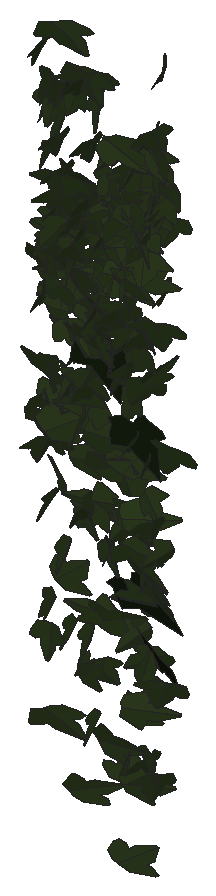
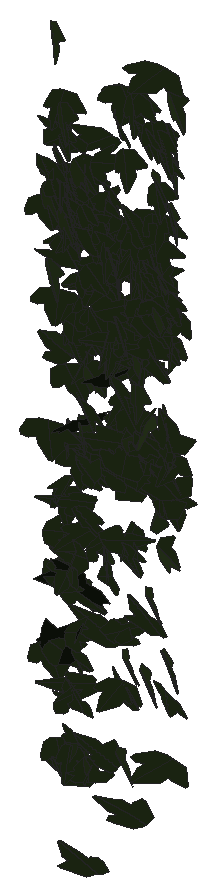
# SketchUp Ruby script. Lengths in millimetres.
U = 1.mm
M = Sketchup.active_model
def pt(a) = Geom::Point3d.new(a.map { |v| v * U })
def face(e, loops, mat)
  f = e.add_face(loops[0].map { |a| pt(a) })
  loops[1..].each { |l| e.add_face(l.map { |a| pt(a) }).erase! }
  f.material = f.back_material = mat if mat
  f
end
# faces: each face lists its corners as indices into pts; further lists are holes
def faces(e, pts, list, mat = nil) = list.each { |f| face(e, (f[0].is_a?(Array) ? f : [f]).map { |l| l.map { |i| pts[i] } }, mat) }
# xy, xz, yz: faces in a plane at the given z, y or x. An outline is a flat list of corners, or four numbers for a rectangle; further outlines are holes
def ring(l) = l.size == 4 ? [[l[0], l[1]], [l[2], l[1]], [l[2], l[3]], [l[0], l[3]]] : l.each_slice(2).to_a
def flat(e, list, mat, &to3) = list.each { |f| face(e, (f[0].is_a?(Array) ? f : [f]).map { |l| ring(l).map { |u, v| to3.(u, v) } }, mat) }
def xy(e, z, list, mat = nil) = flat(e, list, mat) { |x, y| [x, y, z] }
def xz(e, y, list, mat = nil) = flat(e, list, mat) { |x, z| [x, y, z] }
def yz(e, x, list, mat = nil) = flat(e, list, mat) { |y, z| [x, y, z] }
def lines(e, pts, list) = list.each { |a, b| e.add_line(pt(pts[a]), pt(pts[b])) }
# prism: a flat outline (further loops are holes) pulled along v
def prism(e, loops, v, mat = nil)
  f = face(e, loops, mat); d = Geom::Vector3d.new(v.map { |x| x * U })
  f.pushpull(f.normal.samedirection?(d) ? d.length : -d.length)
end
def box(e, o, s, mat = nil) = prism(e, [[o, [o[0] + s[0], o[1], o[2]], [o[0] + s[0], o[1] + s[1], o[2]], [o[0], o[1] + s[1], o[2]]]], [0, 0, s[2]], mat)
def at(x, y, z, deg = 0) = Geom::Transformation.translation(pt([x, y, z])) * Geom::Transformation.rotation(ORIGIN, Z_AXIS, deg.degrees)
def axes(o, x, y, z) = Geom::Transformation.new([*x, 0, *y, 0, *z, 0, *pt(o).to_a, 1])
def part(name) = M.definitions.add(name)
# library, detail: a bought-in or finely detailed component or shape, given as its bounding box
def library(name, o, s) = part(name).tap { |d| box(d.entities, o, s) }
def detail(e, o, s) = box(e.add_group.entities, o, s)
def put(e, d, t, mat = nil) = e.add_instance(d, t).tap { |i| i.material = mat if mat }
def group(e, t, mat = nil) = e.add_group.tap { |g| g.transformation = t; g.material = mat if mat }.entities
root = M.entities
M.materials.add("efeu1").color = [18, 25, 13]
M.materials.add("efeu2").color = [43, 57, 29]
c1 = part("ivyleaf_10")
p = [[0,12.8,-0.8],[-1.5,51.3,-10.9],[-4.9,51,-11.6],[-13.6,26.5,-7.3],[-13.2,15.9,-4.6],[-21.1,19.3,-7.2],
  [-29.5,16.3,-8.3],[-29.2,8.3,-6.2],[-19.7,-9.8,0.5],[-7.6,-13,4],[1,-12.2,5.8],[-0.4,51.1,-11.1],
  [-1.5,51.1,-10.9],[1,-12.4,5.9],[16.9,-12.4,3.5],[35.1,9.1,-5.1],[35,12.9,-6.1],[20.5,16.4,-4.9],
  [15.8,15,-3.8],[15.3,27.6,-7.1],[12.8,31.3,-7.8]]
faces(c1.entities,p,[[0,1,2,3,4,5,6,7,8,9,10],[11,12,0,13,14,15,16,17,18,19,20]],"efeu2")
c2 = part("ivyleaf_9")
p = [[39.1,54.8,31.7],[34.5,51.8,30.2],[-5.3,25.2,17.3],[-17.9,28.3,20.9],[-21.6,21.7,17],[-20.2,4.3,5.3],
  [-22.9,-0.3,2.5],[-17.1,-4,-0.6],[-2,-2.1,-1.2],[-0.7,-15.4,-10.1],[16.6,-22.3,-16.7],[21.1,-15.1,-12.5],
  [32.7,-10.7,-11],[46.1,-1.8,-6.6],[30.8,11.2,3.8]]
faces(c2.entities,p,[[0,1,2,3,4,5,6,7,8,9,10,11,12,13,14]],"efeu1")
put(root,c1,axes([1499.8,1027.3,1054.7],[0.18539,-0.72191,-0.0235],[-0.01929,0.02234,-0.72842],[1.37454,0.09768,-0.00705]))
put(root,c1,axes([1500.7,1029.5,518.1],[-0.35286,-0.6431,0.00823],[-0.00439,-0.0079,-0.66929],[1.22403,-0.18542,-0.00003]))
put(root,c1,axes([1490.9,1042.9,604],[-1.17234,0.16189,0.30669],[0.55873,-0.08938,0.63681],[0.35137,0.68228,0.01065]))
put(root,c1,axes([1501.9,1031.3,972.9],[0.35833,-0.62964,-0.25162],[-0.09136,0.24811,-0.65677],[1.28725,0.19288,0.02343]))
put(root,c1,axes([1493.9,1029.2,766.2],[-1.04653,0.28475,-0.17468],[0.27916,-0.09646,-0.61899],[-0.57121,-0.56884,0.01753]))
put(root,c1,axes([1502.7,1028.3,904.4],[0.33136,-0.59957,-0.27894],[-0.09067,0.27633,-0.62369],[1.25529,0.17823,0.02858]))
put(root,c1,axes([1496.4,1032.2,574.7],[-0.41017,-0.48565,-0.40585],[0.34836,0.36258,-0.53108],[1.15307,-0.2823,0.01608]))
put(root,c1,axes([1505.6,1032.9,304.2],[0.46916,-0.61543,-0.20288],[-0.14756,0.18749,-0.66296],[1.22442,0.25841,-0.00216]))
put(root,c1,axes([1504.6,1018,722.1],[-0.01377,-0.47935,-0.49437],[0.07307,0.49334,-0.47892],[1.30851,-0.03259,0.02154]))
put(root,c1,axes([1509.2,1046.3,787.9],[0.66422,0.37677,-0.38742],[-0.57736,-0.24507,-0.51163],[-0.85118,0.46025,0.04472]))
put(root,c1,axes([1507.2,1040.8,797.6],[1.1056,-0.27653,-0.19393],[-0.31433,0.10397,-0.643],[0.56071,0.60354,0.02192]))
put(root,c1,axes([1493.6,1040.6,538.2],[-0.81421,-0.42933,0.34425],[0.49786,0.22496,0.60565],[-0.92143,0.50092,0.02305]))
put(root,c1,axes([1509.2,1021,1005.8],[0.42926,-0.59634,-0.35365],[-0.15389,0.34673,-0.63624],[1.31052,0.23604,0.04113]))
put(root,c1,axes([1506.3,1041,826],[0.25976,-0.64431,0.12548],[0.02698,-0.12524,-0.6585],[1.24899,0.13671,-0.01187]))
put(root,c1,axes([1495.7,1044.8,513.9],[-0.98982,0.25845,0.41449],[0.69298,-0.19845,0.58062],[0.61968,0.63475,0.01276]))
put(root,c1,axes([1511.6,1032.1,1000.4],[0.67253,-0.44125,-0.43697],[-0.2608,0.43497,-0.55004],[1.15276,0.35584,0.13049]))
put(root,c1,axes([1523.8,1027.1,733.8],[-0.90524,0.162,0.39647],[-0.78739,-0.02057,-0.48794],[-0.2108,-0.61887,0.12]))
put(root,c1,axes([1500,1033.3,573.8],[-0.29107,0.53976,-0.39567],[0.21426,-0.37934,-0.56099],[-1.25557,-0.18986,-0.00401]))
put(root,c1,axes([1499.8,1037.6,258.7],[1.01907,-0.34827,0.22096],[0.35185,-0.12102,-0.63875],[0.7017,0.56647,-0.00062]))
put(root,c1,axes([1508.7,1044.1,775.6],[0.15782,-0.59778,0.32093],[0.14329,-0.31322,-0.60286],[1.28332,0.10849,0.02785]))
put(root,c1,axes([1530.7,1028.5,533.9],[-0.26969,0.05142,0.62374],[-1.13648,0.18037,-0.15053],[-0.35662,-0.61367,0.00802]))
put(root,c1,axes([1522,1016.5,613],[-0.01044,-0.01778,0.68873],[-0.81153,0.54108,0.01057],[-1.02993,-0.42616,-0.01531]))
put(root,c1,axes([1511,1032,448.2],[0.28195,-0.54853,0.36991],[0.13113,-0.36422,-0.56768],[1.25231,0.16164,-0.02384]))
put(root,c1,axes([1511.8,1043.3,947.8],[0.61311,-0.60836,0.03694],[0.05906,-0.02536,-0.68821],[1.15845,0.32327,0.01554]))
put(root,c1,axes([1534,1037.7,559.6],[-0.87151,-0.06403,0.53508],[-0.98256,-0.14922,-0.45968],[0.29409,-0.68828,0.04988]))
put(root,c1,axes([1508,1034.8,980.9],[1.05257,-0.41382,0.16129],[0.23218,-0.10614,-0.69064],[0.81279,0.56623,-0.01158]))
put(root,c1,axes([1517.6,1034.9,930.2],[-0.17866,-0.66963,-0.14527],[0.04485,0.14338,-0.67617],[1.30332,-0.09673,0.00336]))
put(root,c1,axes([1498.7,1045.9,584.6],[0.08546,-0.11336,0.64522],[0.93209,-0.42372,-0.10853],[0.82806,0.48865,0.05557]))
put(root,c1,axes([1520.2,1046.3,816],[1.13958,-0.12566,-0.22355],[-0.4224,0.03057,-0.61164],[0.24454,0.63841,-0.01471]))
put(root,c1,axes([1525.3,1044.3,776.4],[-1.09996,-0.24468,0.20168],[-0.32029,-0.11866,-0.62624],[0.51147,-0.60052,0.04156]))
put(root,c1,axes([1530.5,1045.2,760.8],[0.09658,0.24534,-0.60965],[-0.94481,-0.38635,-0.1968],[-0.81953,0.47432,0.15504]))
put(root,c1,axes([1519.9,1034.9,852.8],[-0.61834,-0.60884,-0.06624],[0.05415,0.05989,-0.69009],[1.16432,-0.32612,-0.00308]))
put(root,c1,axes([1524.9,1032.3,815.5],[-0.53299,-0.48958,0.37395],[-0.15987,-0.37659,-0.55595],[1.16153,-0.27649,0.09508]))
put(root,c1,axes([1522.4,1035.4,886.4],[-0.24969,-0.65979,-0.19016],[0.05073,0.18856,-0.67263],[1.30585,-0.13348,-0.01023]))
put(root,c1,axes([1503.8,1044.7,694.1],[0.63712,-0.3555,-0.47492],[0.6321,-0.33953,0.48826],[-0.93551,-0.47152,0.00647]))
put(root,c1,axes([1521,1046.5,828.4],[0.93213,-0.45924,-0.02017],[-0.01641,0.02029,-0.67134],[0.87472,0.48977,0.0089]))
put(root,c1,axes([1522.5,1052,555.7],[0.13391,0.32415,-0.55107],[-0.22821,-0.53787,-0.3317],[-1.1952,0.13902,0.00159]))
put(root,c1,axes([1528.6,1028,1005],[-0.31275,-0.70047,-0.06187],[0.03535,0.05919,-0.71947],[1.33785,-0.16531,0.00455]))
put(root,c1,axes([1514.5,1025.8,158.1],[-1.01911,-0.25113,-0.44326],[0.79701,0.14926,-0.59045],[0.55219,-0.67892,0.03415]))
put(root,c1,axes([1527.7,1025.4,477.3],[-0.75598,0.56291,0.18241],[0.1514,-0.1669,0.68828],[1.11594,0.40397,0.03019]))
put(root,c1,axes([1523.8,1040.4,380.4],[0.64744,-0.5829,0.20911],[0.2004,-0.18066,-0.6749],[1.16144,0.35611,-0.00012]))
put(root,c1,axes([1530.9,1022.9,882.2],[-1.30455,-0.12976,-0.01894],[0.03596,0.00199,-0.69762],[0.24696,-0.68571,0.00156]))
put(root,c1,axes([1522.2,1034.3,708.9],[0.93875,0.3722,-0.16877],[0.26061,0.09872,0.61791],[0.73284,-0.51189,-0.00355]))
put(root,c1,axes([1516.1,1033.1,578.2],[0.95484,0.21544,-0.38775],[0.61887,0.21954,0.54271],[0.57421,-0.59486,0.05986]))
put(root,c1,axes([1533.4,1030.4,841.8],[0.44181,-0.67517,-0.16839],[-0.05653,0.16773,-0.7135],[1.32314,0.23261,0.02574]))
put(root,c1,axes([1532,1040.4,274.8],[0.53761,-0.63719,0.02041],[0.01527,-0.01877,-0.69699],[1.21322,0.28259,-0.00027]))
put(root,c1,axes([1525,1026.7,1082.6],[-1.11191,-0.24718,-0.35629],[0.67093,0.07738,-0.63175],[0.48059,-0.67991,0.05763]))
put(root,c1,axes([1536.2,1040.6,819.9],[-0.02463,-0.62664,-0.24537],[0.06117,0.24456,-0.62627],[1.27933,-0.02376,0.02522]))
put(root,c1,axes([1537.6,1032.1,608.3],[0.60859,-0.19965,-0.61096],[0.01375,0.68347,-0.21956],[1.22322,0.09165,0.30644]))
put(root,c1,axes([1535,1035.9,608.9],[-0.07522,-0.15495,0.62079],[0.43216,-0.58488,-0.13153],[1.13846,0.21178,0.09095]))
put(root,c1,axes([1524.6,1035.6,341.3],[1.0396,-0.29907,-0.35737],[0.61836,-0.15029,0.62239],[-0.63576,-0.63521,0.02099]))
put(root,c1,axes([1544.5,1034.1,855.4],[-0.6631,-0.57057,-0.12086],[0.10127,0.1091,-0.66844],[1.10537,-0.35227,-0.01126]))
put(root,c1,axes([1545.7,1039.2,651.5],[-0.02642,-0.57456,-0.32341],[0.00271,0.32345,-0.5747],[1.25483,-0.01279,-0.00557]))
put(root,c1,axes([1537.4,1034.7,773.8],[0.09494,-0.32848,0.58836],[0.53964,-0.52497,-0.31713],[1.1634,0.27031,0.09908]))
put(root,c1,axes([1545.1,1032,1002.9],[1.00464,-0.47279,-0.01699],[0.00857,0.03047,-0.70818],[0.90035,0.52726,0.02569]))
put(root,c1,axes([1537.2,1039.8,786.2],[0.44689,-0.45598,0.45044],[0.54075,-0.35595,-0.50845],[1.09345,0.36239,0.06735]))
put(root,c1,axes([1539.2,1036.3,562.9],[0.82694,-0.46873,0.30165],[0.38149,-0.22549,-0.63911],[0.98988,0.47847,-0.00569]))
put(root,c1,axes([1531.3,1048.2,868],[-0.81085,0.12559,0.55668],[0.96511,-0.23535,0.44119],[0.4982,0.66032,0.05137]))
put(root,c1,axes([1527.9,1012.9,553.4],[0.54053,0.23927,-0.69912],[1.03318,0.44057,0.37132],[0.9541,-0.61264,-0.00601]))
put(root,c1,axes([1541.8,1041.8,681.4],[0.02206,-0.16452,-0.62767],[0.05351,-0.62705,0.16488],[-1.23377,-0.03014,-0.00407]))
put(root,c1,axes([1548.7,1026.4,761.8],[-1.09095,0.29702,-0.00692],[0.01299,-0.00187,-0.6456],[-0.56529,-0.57326,-0.00148]))
put(root,c1,axes([1569.1,1034.7,851.9],[-0.85135,0.03746,-0.51049],[-0.96639,0.05308,0.44884],[0.12292,0.67667,-0.00695]))
put(root,c1,axes([1540.9,1026.2,686.4],[0.69343,0.51118,0.17961],[0.1553,0.1622,-0.62718],[-1.01943,0.37242,0.02663]))
put(root,c1,axes([1546.7,1035.6,753.7],[1.36333,-0.04816,-0.04057],[-0.07515,0.01731,-0.7178],[0.09336,0.71727,0.0146]))
put(root,c1,axes([1553.7,1043,619.5],[-0.46303,-0.56355,0.17761],[0.00334,-0.19277,-0.60923],[1.12456,-0.23147,0.07494]))
put(root,c1,axes([1575.7,1016.5,679.1],[-0.20907,0.12575,-0.71735],[-1.14122,0.39611,0.16126],[0.78665,0.60807,0.0433]))
put(root,c1,axes([1555.1,1032.1,822.3],[0.11046,-0.57536,-0.35999],[0.067,0.36337,-0.57509],[1.28996,0.03039,0.0607]))
put(root,c1,axes([1554.1,1017.3,801.8],[-0.38242,-0.51899,-0.34534],[0.22448,0.32463,-0.5565],[1.16501,-0.23291,-0.00613]))
put(root,c1,axes([1553.5,1035.1,837.1],[-0.38893,-0.50261,-0.45725],[0.31106,0.4271,-0.54251],[1.25521,-0.26157,-0.00724]))
put(root,c1,axes([1560.7,1044.9,546.1],[-1.26909,-0.09016,-0.06399],[-0.11863,-0.01655,0.67284],[-0.17378,0.66968,0.00801]))
put(root,c1,axes([1580.9,1036.4,817.5],[0.18752,0.07319,-0.70142],[-1.33632,0.0764,-0.09066],[0.12549,0.70418,0.08274]))
put(root,c1,axes([1571.7,1052.7,449.8],[0.16355,0.11931,0.62257],[-0.65758,-0.51792,0.14695],[1.01147,-0.356,-0.00514]))
put(root,c1,axes([1561.5,1023,1026.5],[-0.20659,-0.66403,-0.28612],[0.05387,0.2852,-0.67263],[1.37505,-0.11094,-0.01664]))
put(root,c1,axes([1564.3,1044.4,439.9],[1.02347,-0.26423,-0.22129],[-0.36127,0.11524,-0.59889],[0.5475,0.56998,0.01849]))
put(root,c1,axes([1541.6,1047,433.4],[0.38552,-0.20956,0.64495],[1.04402,-0.3451,-0.28442],[0.75879,0.58129,0.06365]))
put(root,c1,axes([1561.7,1033.1,859.6],[-0.23255,-0.5641,-0.39116],[0.17698,0.38004,-0.57712],[1.2944,-0.15331,0.00863]))
put(root,c1,axes([1561.9,1023.2,451],[-0.12029,-0.46032,-0.55569],[0.2039,0.54565,-0.46418],[1.3581,-0.12269,0.02047]))
put(root,c1,axes([1583,1022.9,594.5],[0.60007,-0.08677,-0.62442],[-1.14728,0.16283,-0.32702],[0.35114,0.68029,-0.00137]))
put(root,c1,axes([1561.5,1047.9,156.4],[0.56253,-0.60579,0.15281],[0.11407,-0.14077,-0.674],[1.18357,0.30149,-0.00767]))
put(root,c1,axes([1558.3,1042.1,585.8],[0.05227,-0.20104,0.6447],[0.53224,-0.58393,-0.194],[1.16989,0.27464,0.05946]))
put(root,c1,axes([1569.1,1043.4,737.5],[0.5169,-0.55572,-0.21183],[-0.08883,0.21224,-0.61663],[1.12838,0.27128,0.04849]))
put(root,c1,axes([1563.4,1033.8,279.9],[0.65216,-0.53548,0.23816],[0.23795,-0.20274,-0.63572],[1.0897,0.36474,-0.00371]))
put(root,c1,axes([1563.5,1024.6,1035.1],[-1.28275,0.13808,-0.21923],[0.36577,-0.1433,-0.68112],[-0.33069,-0.69412,0.097]))
put(root,c1,axes([1586.2,1024,720],[-0.17264,0.19805,-0.6082],[-0.78606,0.45091,0.20843],[0.92953,0.4181,0.0633]))
put(root,c1,axes([1572.9,1023.6,1034.7],[-1.14612,-0.37852,-0.095],[0.13074,0.06915,-0.71095],[0.73114,-0.60572,-0.02179]))
put(root,c1,axes([1582.8,1033.3,312.1],[0.30139,0.2977,0.55175],[-0.46813,-0.49395,0.33711],[1.09752,-0.29244,-0.00773]))
put(root,c1,axes([1577.6,1042.1,656.2],[0.80538,-0.44683,-0.21759],[-0.26289,0.16877,-0.61523],[0.9086,0.4449,0.01486]))
put(root,c1,axes([1575.8,1022.1,948.2],[-0.21874,-0.69555,-0.19295],[0.06102,0.19027,-0.70498],[1.37241,-0.11932,0.00059]))
put(root,c1,axes([1577.7,1028.8,668.5],[0.06164,0.65673,-0.17983],[-0.00751,0.18021,0.65741],[1.29588,-0.03019,0.01236]))
put(root,c1,axes([1558.5,1024.9,69.6],[-0.5456,-0.24816,0.55822],[0.76562,0.38737,0.3788],[-0.87497,0.4937,-0.01662]))
put(root,c1,axes([1585.5,1050,752.8],[0.21364,0.27553,0.57456],[-0.44237,-0.52551,0.29741],[1.12918,-0.258,0.00781]))
put(root,c1,axes([1580.2,1011.5,705],[0.16966,-0.12975,0.77518],[-0.50762,0.72886,0.15267],[-1.40708,-0.27859,0.03839]))
put(root,c1,axes([1560.2,1031.6,228.6],[0.66865,-0.39385,-0.43661],[0.53033,-0.33635,0.52764],[-0.98544,-0.44825,-0.01229]))
put(root,c1,axes([1594.1,1030.8,714.1],[-1.00159,-0.00248,0.43532],[-0.82848,0.00979,-0.52619],[-0.00825,-0.68291,-0.00912]))
put(root,c1,axes([1567.1,1029.3,678.6],[-1.01759,0.16729,-0.30873],[0.55304,-0.10493,-0.56011],[-0.37518,-0.60842,0.01171]))
put(root,c1,axes([1582.6,1031.1,805],[0.37263,-0.55272,-0.3456],[-0.06807,0.3512,-0.58194],[1.23878,0.18556,0.07198]))
put(root,c1,axes([1583.9,1036.5,819.8],[0.24918,-0.64723,-0.20686],[-0.09331,0.20112,-0.66029],[1.28982,0.13959,-0.00781]))
put(root,c1,axes([1577.1,1017.7,621],[-0.44987,-0.46721,-0.47243],[0.38797,0.42625,-0.52354],[1.20356,-0.31204,-0.00782]))
put(root,c1,axes([1557,1028.9,512.9],[0.30454,-0.0032,-0.62674],[1.18554,-0.07054,0.1594],[-0.13158,-0.64298,-0.01437]))
put(root,c1,axes([1581.7,1039.4,697],[-0.01748,-0.54484,-0.35414],[0.15669,0.35035,-0.54114],[1.22678,-0.05251,0.06407]))
put(root,c1,axes([1558.9,1037.7,712.9],[0.25393,0.0934,0.70297],[1.01572,0.4578,-0.16212],[-0.88874,0.54989,0.01557]))
put(root,c1,axes([1577.4,1032.7,241.6],[-0.74519,-0.42383,-0.35869],[0.4943,0.24813,-0.5767],[0.934,-0.46947,0.01902]))
put(root,c1,axes([1586.8,1031.3,771.2],[0.85412,-0.44902,-0.14413],[-0.18505,0.10658,-0.63481],[0.87824,0.45915,0.00641]))
put(root,c1,axes([1576.3,1034,1000.6],[0.68285,-0.49456,0.39986],[0.50036,-0.3027,-0.61029],[1.10214,0.44384,0.02932]))
put(root,c1,axes([1589.6,1038.8,827.1],[-0.05524,-0.59884,-0.35837],[0.06368,0.35707,-0.59938],[1.32668,-0.04207,0.01385]))
put(root,c2,axes([1577.3,1039.1,665.8],[-0.16328,-0.76793,-0.21996],[0.08419,0.21632,-0.77247],[1.51797,-0.0946,0.01918]))
put(root,c1,axes([1590.3,1037.7,704.2],[0.127,-0.4912,-0.42817],[0.18264,0.43312,-0.48192],[1.22663,-0.01363,0.11609]))
put(root,c1,axes([1595.1,1034.3,851.6],[-0.49886,-0.59598,0.10222],[0.01951,-0.11577,-0.64872],[1.15067,-0.25642,0.05531]))
put(root,c1,axes([1596.6,1037.2,842],[-1.21227,0.21757,0.00256],[-0.00459,0.00085,-0.6731],[-0.41408,-0.63697,-0.00003]))
put(root,c1,axes([1578.6,1046.1,396],[0.50834,-0.27729,0.5144],[0.85699,-0.26284,-0.37549],[0.7089,0.51659,0.08506]))
put(root,c1,axes([1597,1030.5,904.2],[0.82566,-0.53894,-0.01151],[-0.01869,0.00686,-0.69185],[1.02578,0.43392,-0.00335]))
put(root,c1,axes([1602.1,1026.2,413],[0.19081,-0.47514,-0.43178],[-0.10468,0.42905,-0.4849],[1.21741,0.11136,0.02598]))
put(root,c1,axes([1596,1029.3,802.1],[-1.11503,-0.2297,-0.17629],[0.35453,0.00562,-0.62638],[0.42189,-0.6118,0.06044]))
put(root,c1,axes([1596.4,1032.1,897.5],[0.35091,0.64508,-0.10771],[-0.03648,-0.10653,-0.67083],[-1.24418,0.18506,-0.01071]))
put(root,c1,axes([1583.8,1036.4,875.2],[-0.26012,0.10033,-0.66092],[0.78706,-0.51733,-0.16405],[-0.99961,-0.43343,0.04281]))
put(root,c1,axes([1601.5,1040.6,940.5],[-0.08904,-0.25073,0.67973],[0.22027,-0.67498,-0.24101],[1.36116,0.09283,0.08347]))
put(root,c1,axes([1575,1040.6,529.7],[0.02076,-0.01962,0.78333],[1.45357,-0.17483,-0.01501],[0.33331,0.76365,0.01669]))
put(root,c1,axes([1611.9,1037.9,730.3],[-0.79341,-0.46521,0.2029],[-0.23689,-0.16084,-0.62452],[0.93644,-0.43484,0.01392]))
put(root,c1,axes([1608.3,1045.3,795],[-0.36114,-0.57246,0.28821],[-0.0034,-0.3001,-0.59726],[1.21978,-0.17032,0.08366]))
put(root,c1,axes([1608.7,1018.6,682],[0.48866,-0.43077,-0.48205],[-0.1019,0.50272,-0.47777],[1.22615,0.21346,0.15241]))
put(root,c1,axes([1601.4,1052.5,428.6],[-0.18795,-0.07197,0.66743],[0.38648,-0.64621,-0.03964],[1.21776,0.19398,0.11559]))
put(root,c1,axes([1607,1035.1,861],[1.13876,0.24749,-0.13382],[-0.22788,-0.06059,-0.64743],[-0.48456,0.61012,-0.01001]))
put(root,c1,axes([1590.6,1031.5,305.6],[-0.83286,-0.17389,0.55924],[0.97859,0.22014,0.4708],[-0.53361,0.67512,-0.00947]))
put(root,c1,axes([1610.4,1045.3,842.2],[1.22837,0.09393,-0.12404],[-0.24889,0.04074,-0.64963],[-0.16044,0.65597,0.05811]))
put(root,c1,axes([1616.2,1039.9,873.8],[-0.29148,-0.62134,0.23451],[-0.09184,-0.22961,-0.63989],[1.26062,-0.1604,0.00761]))
put(root,c1,axes([1595.1,1023.7,514.5],[-0.78149,-0.26972,0.49443],[0.7863,0.27161,0.49128],[-0.72851,0.58249,-0.00013]))
put(root,c1,axes([1611.2,1029,727.2],[-0.52791,-0.54194,-0.30528],[0.22476,0.2823,-0.60844],[1.16228,-0.30074,-0.021]))
put(root,c1,axes([1590.3,1034.6,140.3],[-0.50859,-0.01678,0.64432],[1.22654,0.0039,0.26739],[-0.01909,0.69753,0.01401]))
put(root,c1,axes([1588.2,1021,560.6],[-0.24751,-0.0602,-0.75149],[1.40686,0.13965,-0.13911],[0.28191,-0.74977,0.03443]))
put(root,c1,axes([1628.3,1035.7,457.2],[0.65096,-0.28019,-0.48652],[-0.71857,0.30684,-0.44215],[0.79082,0.50945,-0.00128]))
put(root,c1,axes([1618,1033.9,651.4],[0.03904,-0.62852,0.23191],[0.02839,-0.23153,-0.62881],[1.27471,0.02441,0.0069]))
put(root,c1,axes([1616.1,1028,770],[-1.19793,0.18675,-0.06649],[0.11656,-0.02732,-0.65649],[-0.35883,-0.63234,0.00873]))
put(root,c1,axes([1603.1,1025.1,780.2],[-0.15258,-0.27202,-0.62845],[0.85624,0.45611,-0.25481],[0.98257,-0.43971,0.12447]))
put(root,c1,axes([1601.8,1053,524.8],[-0.37785,-0.02629,0.61256],[1.01785,-0.32229,0.1595],[0.57063,0.55747,0.1211]))
put(root,c1,axes([1615.5,1046.8,122.5],[0.01185,0.03633,-0.6792],[-0.02516,-0.67909,-0.03644],[-1.29425,0.01353,-0.00551]))
put(root,c1,axes([1620.3,1043.3,610.9],[0.93259,-0.44367,0.04357],[0.06918,-0.02476,-0.661],[0.84563,0.49132,0.00603]))
put(root,c1,axes([1630.3,1032.4,705.8],[-0.46031,-0.56119,0.25106],[-0.19425,-0.22939,-0.61109],[1.15383,-0.2625,-0.00272]))
put(root,c1,axes([1628.5,1041.2,927.4],[-0.14831,-0.68304,0.24413],[-0.02139,-0.24437,-0.6873],[1.38034,-0.07717,0.01558]))
put(root,c1,axes([1620.5,1035.4,106.4],[0.872,0.44433,-0.12968],[0.16828,0.09509,0.63821],[0.86471,-0.46658,0.00658]))
put(root,c1,axes([1623.5,1042,778.9],[-0.057,-0.53898,0.41742],[0.22776,-0.41549,-0.5279],[1.2773,0.05004,0.11276]))
put(root,c1,axes([1633.9,1023.3,503.9],[0.92349,-0.20979,0.38706],[-0.67924,0.14985,0.52863],[-0.49063,-0.60234,-0.0033]))
put(root,c1,axes([1630.6,1031.3,529.1],[-1.27702,-0.21035,0.00415],[-0.00628,-0.00333,-0.70318],[0.40037,-0.67099,0.00219]))
put(root,c1,axes([1625.4,1030.3,667.2],[0.15765,-0.33916,-0.69143],[0.22718,0.69267,-0.32546],[1.448,-0.07175,0.12634]))
put(root,c1,axes([1630.7,1028.9,927.1],[0.17629,-0.58298,-0.4239],[-0.06146,0.4236,-0.58962],[1.37045,0.09399,0.02809]))
put(root,c1,axes([1620.4,1014.8,863.1],[-0.21105,-0.54035,-0.57495],[0.62671,0.49593,-0.52959],[1.36463,-0.31132,0.1543]))
put(root,c1,axes([1652.1,1031.7,352.5],[-0.54346,-0.02384,0.59598],[-1.13047,-0.04877,-0.28654],[0.10331,-0.65906,-0.00035]))
put(root,c1,axes([1608.6,1023.9,774.9],[0.60904,0.18948,0.5792],[0.87654,0.35322,-0.37001],[-0.75953,0.55957,0.03743]))
put(root,c1,axes([1641.3,1031.2,847.5],[0.91555,0.23471,-0.44909],[-0.81972,-0.13683,-0.53288],[-0.50806,0.64372,0.05048]))
put(root,c1,axes([1627.8,1031.9,837.7],[1.25376,0.21686,-0.05702],[-0.10247,-0.01879,-0.69354],[-0.41427,0.66096,-0.00101]))
put(root,c1,axes([1634.3,1045.5,300],[-0.17237,-0.22912,0.6866],[0.08509,-0.69241,-0.22516],[1.37495,0.01413,0.10001]))
put(root,c1,axes([1616.1,1015.7,959.5],[0.67494,0.36615,0.48682],[0.59072,0.37609,-0.50897],[-0.99755,0.47044,0.02799]))
put(root,c1,axes([1614.4,1040.9,-10.5],[0.94168,0.04999,-0.4406],[0.83571,0.03671,0.49727],[0.11753,-0.66151,-0.0057]))
put(root,c1,axes([1628.9,1043.6,877.2],[1.08224,-0.37135,0.07596],[0.20961,0.03082,-0.67376],[0.69026,0.57287,0.08549]))
put(root,c1,axes([1638.8,1025,571.4],[0.1026,-0.58364,-0.27077],[-0.03075,0.2704,-0.58607],[1.22412,0.05571,0.00797]))
put(root,c1,axes([1642.4,1025.4,871.3],[0.67494,-0.5377,-0.25259],[-0.26365,0.21122,-0.64412],[1.09948,0.38073,0.0006]))
put(root,c1,axes([1640.2,1036.6,914.3],[-1.12677,-0.36167,0.04779],[0.06779,-0.14797,-0.67855],[0.69099,-0.57524,0.1445]))
put(root,c1,axes([1634.7,1042.3,896.8],[0.97968,-0.43525,0.05594],[0.12631,-0.00802,-0.67311],[0.82558,0.51772,0.0366]))
put(root,c1,axes([1639.1,1043.8,713],[-0.10632,-0.45061,0.49221],[0.13847,-0.4951,-0.445],[1.26248,0.01636,0.09026]))
put(root,c1,axes([1642.2,1034.9,845.7],[-0.45189,-0.60996,0.18085],[0.03528,-0.19958,-0.64881],[1.21031,-0.22192,0.08644]))
put(root,c1,axes([1649.2,1036.6,641.5],[-0.81185,-0.46754,0.19759],[-0.259,-0.1433,-0.63288],[0.93066,-0.44773,-0.00377]))
put(root,c1,axes([1656,1048.5,274],[-0.57591,-0.29674,0.48488],[-0.58642,-0.37599,-0.42239],[0.9092,-0.43047,0.03469]))
put(root,c1,axes([1645.6,1032.9,837.3],[0.358,-0.58742,-0.25252],[-0.08438,0.2506,-0.61599],[1.21397,0.19065,0.03165]))
put(root,c1,axes([1646.1,1046.5,860.8],[-0.07304,-0.67635,-0.02533],[0.00025,0.02536,-0.67743],[1.28812,-0.03836,-0.0013]))
put(root,c1,axes([1644.2,1043.6,876.4],[0.38259,-0.63737,-0.12925],[0.03553,0.14088,-0.6657],[1.23721,0.19305,0.05908]))
put(root,c1,axes([1629,1025.9,527.8],[1.24572,0.19171,-0.32038],[0.58553,0.08937,0.68204],[0.40257,-0.72324,-0.00064]))
put(root,c1,axes([1645,1030.4,685.7],[1.01155,-0.32105,-0.18696],[-0.15507,0.21767,-0.60539],[0.68986,0.51968,0.13806]))
put(root,c1,axes([1644.7,1040.8,133.1],[-0.33608,-0.59656,-0.31248],[0.14971,0.30256,-0.62207],[1.27292,-0.19309,-0.00934]))
put(root,c2,axes([1631.2,1033.4,581.7],[0.08904,-0.74995,-0.27279],[-0.02536,0.27249,-0.7514],[1.51858,0.04853,0.00345]))
put(root,c1,axes([1634.9,1035.5,197],[1.10271,-0.27175,-0.14039],[0.24364,-0.05766,0.63996],[-0.5287,-0.59337,0.0021]))
put(root,c1,axes([1633.6,1021.4,424.5],[-0.64119,-0.36166,-0.53534],[0.78985,0.34156,-0.49192],[0.94232,-0.53238,0.04807]))
put(root,c1,axes([1652,1039.8,892.1],[-0.98722,-0.43226,0.04725],[-0.0646,-0.03307,-0.67521],[0.82506,-0.51981,0.00367]))
put(root,c1,axes([1646.8,1054.3,207.6],[-0.25028,0.04158,0.65408],[0.21895,-0.65529,0.06479],[1.22799,0.12531,0.12176]))
put(root,c1,axes([1650.3,1034.8,844.2],[0.01058,-0.60267,-0.36624],[0.14374,0.36465,-0.59891],[1.33446,-0.0345,0.06741]))
put(root,c1,axes([1640.8,1043.7,380.8],[-0.05141,0.02299,0.68133],[0.63164,-0.59516,0.03324],[1.13331,0.33275,0.01238]))
put(root,c1,axes([1650.4,1024.3,714.6],[-0.26941,-0.58604,-0.38884],[0.22259,0.3715,-0.60248],[1.31989,-0.18227,0.02224]))
put(root,c1,axes([1658.8,1025.5,705.8],[-0.86507,0.48299,-0.05741],[-0.11072,0.02403,0.66273],[0.91905,0.45751,0.0258]))
put(root,c1,axes([1647.3,1021.8,829.2],[-0.20772,-0.47043,-0.50662],[0.48104,0.45023,-0.47252],[1.22469,-0.25663,0.09967]))
put(root,c2,axes([1627.9,1035.9,365.7],[-0.12894,-0.1757,-0.75335],[1.37251,0.25927,-0.12532],[0.53267,-0.71057,0.14055]))
put(root,c1,axes([1649.7,1022.7,844.1],[-0.32381,0.63679,-0.08319],[0.03174,-0.08165,-0.65911],[-1.22183,-0.17088,0.00493]))
put(root,c1,axes([1649,1030.4,250.4],[1.00673,-0.38562,0.0331],[-0.04722,0.02216,0.6546],[-0.7351,-0.52954,0.00329]))
put(root,c1,axes([1651.4,1042,873.2],[1.21049,-0.21604,-0.00368],[-0.00646,0.00146,-0.67172],[0.41117,0.63604,0.0003]))
put(root,c1,axes([1654.4,1035.3,374],[-0.97802,0.41527,0.00716],[-0.01075,0.0044,-0.6607],[-0.79039,-0.51391,0.00013]))
put(root,c1,axes([1637.2,1035,398.9],[-0.42421,0.22834,-0.63439],[0.88063,-0.43418,-0.31885],[-0.93333,-0.51344,-0.01251]))
put(root,c1,axes([1653.8,1025.6,817.7],[0.77003,0.5108,-0.1252],[-0.15122,-0.09677,-0.65162],[-0.98944,0.41232,0.00216]))
put(root,c1,axes([1656.3,1041.2,897.5],[0.38602,-0.61472,-0.22205],[0.14503,0.25315,-0.63122],[1.23544,0.16236,0.14348]))
put(root,c1,axes([1633.1,1030.6,102.1],[0.40282,-0.02533,-0.6096],[1.15673,-0.04773,0.21301],[-0.10165,-0.64353,0.0082]))
put(root,c1,axes([1646.8,1034.5,144.2],[-0.34224,0.35131,-0.52353],[0.42904,-0.47259,-0.39456],[-1.1206,-0.28823,0.00882]))
put(root,c1,axes([1661.5,1032.5,984.8],[0.07903,-0.67012,-0.24624],[0.00231,0.24672,-0.67122],[1.35874,0.03856,0.01547]))
put(root,c1,axes([1654.4,1032,493.8],[0.07784,0.65698,0.11134],[0.00246,0.11148,-0.65823],[-1.26819,0.04054,0.00556]))
put(root,c2,axes([1668,1041.9,264.2],[0.46516,-0.54795,0.47861],[-0.30293,0.4524,0.59921],[-1.35111,-0.29008,0.03043]))
put(root,c1,axes([1649.3,1029.4,785.8],[1.37322,0.03371,-0.16606],[0.31344,0.03136,0.72195],[0.07587,-0.73973,0.02304]))
put(root,c1,axes([1661.8,1021.2,555.7],[0.22657,-0.52024,-0.41216],[0.00898,0.41939,-0.528],[1.26316,0.09034,0.07768]))
put(root,c1,axes([1638.6,1023.3,464.5],[0.34965,-0.1444,-0.69529],[1.15442,0.40536,0.07609],[0.70279,-0.59402,0.22094]))
put(root,c1,axes([1654.3,1042.5,921.1],[-0.38163,0.24162,-0.60735],[0.26418,-0.60506,-0.28654],[-1.21565,-0.20734,0.1284]))
put(root,c1,axes([1665.9,1022.3,465.2],[-0.44723,-0.64818,-0.11921],[0.06954,0.11355,-0.68945],[1.25238,-0.23777,-0.00429]))
put(root,c1,axes([1669.6,1031.9,921.3],[0.5629,-0.57193,-0.26548],[-0.2027,0.24371,-0.64368],[1.1828,0.31395,0.01603]))
put(root,c1,axes([1644.7,1014.6,215.3],[0.02989,-0.16133,-0.69699],[1.15419,0.37285,-0.07264],[0.72234,-0.58909,0.14491]))
put(root,c1,axes([1670.3,1031.4,898.2],[1.16737,-0.23963,-0.19798],[-0.34991,0.07347,-0.65852],[0.47701,0.64033,0.00147]))
put(root,c1,axes([1674.2,1029.2,351.5],[-1.14528,0.26805,-0.09464],[-0.17988,0.0203,0.65847],[0.51024,0.60882,0.01971]))
put(root,c1,axes([1672.9,1042.2,775.8],[0.15683,-0.64908,-0.2337],[-0.09218,0.22934,-0.65404],[1.30972,0.09387,-0.01805]))
put(root,c1,axes([1673.4,1027.1,959.5],[0.86591,-0.40858,-0.34243],[-0.25723,0.34708,-0.59369],[0.98145,0.45145,0.14652]))
put(root,c1,axes([1672.3,1044.4,881.5],[-0.06497,-0.68527,0.01798],[0.003,-0.01808,-0.68611],[1.30464,-0.03408,0.00247]))
put(root,c1,axes([1677.2,1042.6,559.3],[-1.31218,-0.12038,0.12223],[-0.22651,-0.02894,-0.69985],[0.23515,-0.69961,0.00792]))
put(root,c1,axes([1674.3,1025.3,125.7],[-0.61472,-0.61615,0.01228],[-0.00794,-0.01167,-0.69568],[1.17287,-0.32301,0.00173]))
put(root,c1,axes([1673.8,1027.4,730.8],[-1.1317,-0.30584,-0.02832],[0.04703,0.01388,-0.66867],[0.58267,-0.59514,-0.00104]))
put(root,c1,axes([1672.1,1042.3,422.7],[-0.02708,-0.19416,0.63171],[0.07965,-0.63086,-0.19296],[1.25526,0.03584,0.02587]))
put(root,c1,axes([1665,1025.5,659.5],[-0.0302,-0.60564,0.37816],[0.12847,0.37529,0.60387],[-1.3528,0.04916,0.0489]))
put(root,c1,axes([1676.7,1045.9,864.9],[-0.87515,-0.47966,0.11029],[-0.00808,-0.14707,-0.6573],[0.93668,-0.44942,0.09737]))
put(root,c1,axes([1672.2,1019.7,994],[-0.49578,-0.60194,-0.31695],[0.27178,0.28344,-0.65568],[1.26587,-0.29661,0.01664]))
put(root,c1,axes([1655.4,1031.5,956.3],[1.03307,0.04361,0.4176],[0.79406,0.02047,-0.54446],[-0.08956,0.68455,-0.01032]))
put(root,c1,axes([1678.7,1042,912.9],[0.94214,-0.39965,-0.24477],[-0.20857,0.24744,-0.62566],[0.8672,0.4937,0.11544]))
put(root,c1,axes([1686.4,1027.7,251.9],[-0.92304,-0.44035,0.12962],[-0.16639,-0.0965,-0.65496],[0.85763,-0.49265,0.01243]))
put(root,c1,axes([1683.1,1023.2,1084.4],[0.1695,-0.59947,-0.38097],[-0.05374,0.38066,-0.60559],[1.35074,0.09037,0.02371]))
